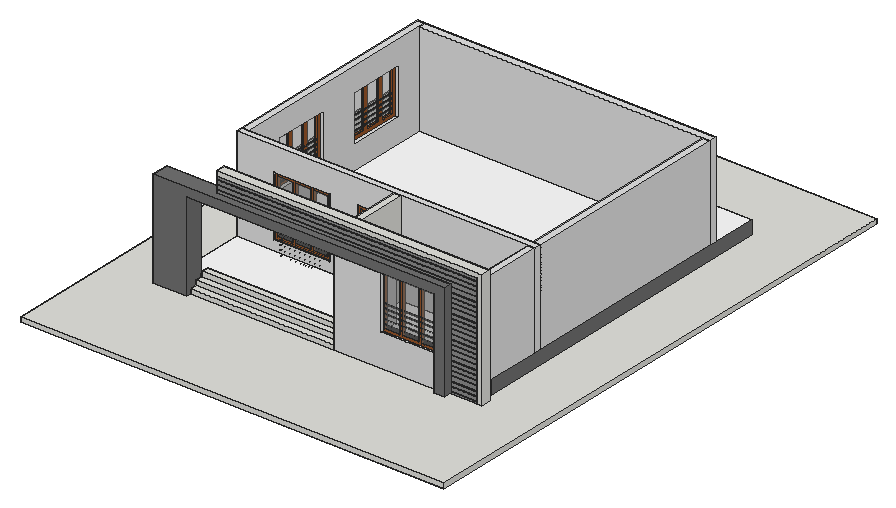
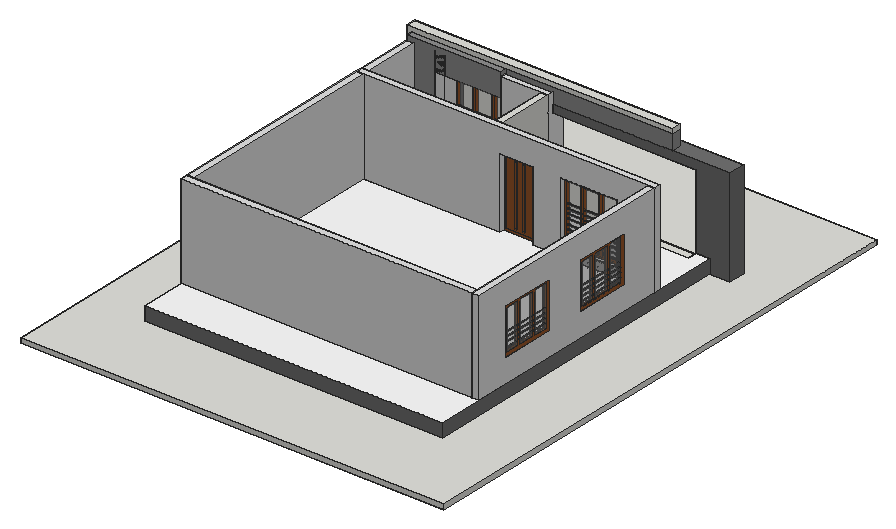
# SketchUp Ruby script. Lengths in inches.
U = 1.inch
M = Sketchup.active_model
def pt(a) = Geom::Point3d.new(a.map { |v| v * U })
def face(e, loops, mat)
  f = e.add_face(loops[0].map { |a| pt(a) })
  loops[1..].each { |l| e.add_face(l.map { |a| pt(a) }).erase! }
  f.material = f.back_material = mat if mat
  f
end
# faces: each face lists its corners as indices into pts; further lists are holes
def faces(e, pts, list, mat = nil) = list.each { |f| face(e, (f[0].is_a?(Array) ? f : [f]).map { |l| l.map { |i| pts[i] } }, mat) }
# xy, xz, yz: faces in a plane at the given z, y or x. An outline is a flat list of corners, or four numbers for a rectangle; further outlines are holes
def ring(l) = l.size == 4 ? [[l[0], l[1]], [l[2], l[1]], [l[2], l[3]], [l[0], l[3]]] : l.each_slice(2).to_a
def flat(e, list, mat, &to3) = list.each { |f| face(e, (f[0].is_a?(Array) ? f : [f]).map { |l| ring(l).map { |u, v| to3.(u, v) } }, mat) }
def xy(e, z, list, mat = nil) = flat(e, list, mat) { |x, y| [x, y, z] }
def xz(e, y, list, mat = nil) = flat(e, list, mat) { |x, z| [x, y, z] }
def yz(e, x, list, mat = nil) = flat(e, list, mat) { |y, z| [x, y, z] }
def lines(e, pts, list) = list.each { |a, b| e.add_line(pt(pts[a]), pt(pts[b])) }
# prism: a flat outline (further loops are holes) pulled along v
def prism(e, loops, v, mat = nil)
  f = face(e, loops, mat); d = Geom::Vector3d.new(v.map { |x| x * U })
  f.pushpull(f.normal.samedirection?(d) ? d.length : -d.length)
end
def box(e, o, s, mat = nil) = prism(e, [[o, [o[0] + s[0], o[1], o[2]], [o[0] + s[0], o[1] + s[1], o[2]], [o[0], o[1] + s[1], o[2]]]], [0, 0, s[2]], mat)
def at(x, y, z, deg = 0) = Geom::Transformation.translation(pt([x, y, z])) * Geom::Transformation.rotation(ORIGIN, Z_AXIS, deg.degrees)
def axes(o, x, y, z) = Geom::Transformation.new([*x, 0, *y, 0, *z, 0, *pt(o).to_a, 1])
def part(name) = M.definitions.add(name)
# library, detail: a bought-in or finely detailed component or shape, given as its bounding box
def library(name, o, s) = part(name).tap { |d| box(d.entities, o, s) }
def detail(e, o, s) = box(e.add_group.entities, o, s)
def put(e, d, t, mat = nil) = e.add_instance(d, t).tap { |i| i.material = mat if mat }
def group(e, t, mat = nil) = e.add_group.tap { |g| g.transformation = t; g.material = mat if mat }.entities
root = M.entities
M.materials.add("[Color M00]").color = [255, 255, 255]
M.materials.add("[Color M01]").color = [226, 226, 226]
M.materials.add("[Color M04]").color = [142, 142, 142]
M.materials.add("[Color M05]").color = [114, 114, 114]
M.materials.add("[Metal Silver]").color = [234, 233, 238]
M.materials.add("[Translucent Glass Gray]").color = [128, 128, 128]
M.materials["[Translucent Glass Gray]"].alpha = 0.5
M.materials.add("[Wood Cherry Original]").color = [152, 86, 42]
c1 = part("Group\#18")
prism(c1.entities,[[[0,1.11,0.71],[0,1.125,0.5625],[0,1.11,0.42],[0,1.05,0.28],[0,0.96,0.16],[0,0.84,0.08],[0,0.71,0.02],[0,0.5625,0],[0,0.42,0.02],[0,0.28,0.08],[0,0.16,0.16],[0,0.08,0.28],[0,0.02,0.42],[0,0,0.5625],[0,0.02,0.71],[0,0.08,0.84],[0,0.16,0.96],[0,0.28,1.05],[0,0.42,1.11],[0,0.5625,1.125],[0,0.71,1.11],[0,0.84,1.05],[0,0.96,0.96],[0,1.05,0.84]]],[64,0,0])
c2 = part("Group\#25")
prism(c2.entities,[[[0.28,64,0.08],[0.16,64,0.16],[0.08,64,0.28],[0.02,64,0.42],[0,64,0.5625],[0.02,64,0.71],[0.08,64,0.84],[0.16,64,0.96],[0.28,64,1.05],[0.42,64,1.11],[0.5625,64,1.125],[0.71,64,1.11],[0.84,64,1.05],[0.96,64,0.96],[1.05,64,0.84],[1.11,64,0.71],[1.125,64,0.5625],[1.11,64,0.42],[1.05,64,0.28],[0.96,64,0.16],[0.84,64,0.08],[0.71,64,0.02],[0.5625,64,0],[0.42,64,0.02]]],[0,-64,0])
c3 = part("Group\#16")
prism(c3.entities,[[[0,2,23.9375],[0,2,22.2],[0,0.74,22.2],[0,0.74,1.74],[0,2,1.74],[0,2,0],[0,0,0],[0,0,23.9375]]],[1.1875,0,0])
c4 = part("Group\#30")
prism(c4.entities,[[[0.15,64,0.15],[0.07,64,0.25],[0.02,64,0.37],[0,64,0.5],[0.02,64,0.63],[0.07,64,0.75],[0.15,64,0.85],[0.25,64,0.93],[0.37,64,0.98],[0.5,64,1],[0.63,64,0.98],[0.75,64,0.93],[0.85,64,0.85],[0.93,64,0.75],[0.98,64,0.63],[1,64,0.5],[0.98,64,0.37],[0.93,64,0.25],[0.85,64,0.15],[0.75,64,0.07],[0.63,64,0.02],[0.5,64,0],[0.37,64,0.02],[0.25,64,0.07]]],[0,-64,0])
g1 = group(root,at(0,0,0))
box(g1,[0,0,0],[542.875,691.875,6])
g2 = group(root,at(47.33,167.375,6),"[Color M05]")
xy(g2,0,[[38,-8,38,420,420,420,420,3,56,3,56,-8]])
xy(g2,18,[[38,-8,56,-8,56,3,420,3,420,420,38,420]],"[Color M00]")
xz(g2,-8,[[38,0,56,18]])
xz(g2,3,[[56,0,420,18]])
xz(g2,420,[[38,0,420,18]])
yz(g2,38,[[-8,0,420,18]])
yz(g2,56,[[-8,0,3,18]])
yz(g2,420,[[3,0,420,18]])
g3 = group(root,at(287.33,143.375,6),"[Color M01]")
xy(g3,0,[[0,0,144,24]])
xy(g3,42,[[60,0,131.9,24]])
xy(g3,114,[[0,0,60,12],[131.9,0,144,12]])
xy(g3,138,[[0,12,60,24],[131.9,12,144,24]])
xz(g3,0,[[0,0,144,0,144,114,131.9,114,131.9,42,60,42,60,114,0,114]])
xz(g3,12,[[0,114,60,138],[131.9,114,144,138]])
xz(g3,24,[[0,0,0,138,60,138,60,42,131.9,42,131.9,138,144,138,144,0]])
yz(g3,0,[[0,0,0,114,12,114,12,138,24,138,24,0]])
yz(g3,60,[[0,42,24,42,24,138,12,138,12,114,0,114]])
yz(g3,131.9,[[0,42,0,114,12,114,12,138,24,138,24,42]])
yz(g3,144,[[0,0,24,0,24,138,12,138,12,114,0,114]])
g4 = group(root,at(287.33,147.375,6),"[Color M04]")
xy(g4,0,[[144,0,180,20]])
xy(g4,2,[[144,0,180,0.5]])
xy(g4,3,[[144,0,180,0.5]])
xy(g4,8,[[144,0,180,0.5]])
xy(g4,9,[[144,0,180,0.5]])
xy(g4,14,[[144,0,180,0.5]])
xy(g4,15,[[144,0,180,0.5]])
xy(g4,20,[[144,0,180,0.5]])
xy(g4,21,[[144,0,180,0.5]])
xy(g4,26,[[144,0,180,0.5]])
xy(g4,27,[[144,0,180,0.5]])
xy(g4,32,[[144,0,180,0.5]])
xy(g4,33,[[144,0,180,0.5]])
xy(g4,38,[[144,0,180,0.5]])
xy(g4,39,[[144,0,180,0.5]])
xy(g4,44,[[144,0,180,0.5]])
xy(g4,45,[[144,0,180,0.5]])
xy(g4,50,[[144,0,180,0.5]])
xy(g4,51,[[144,0,180,0.5]])
xy(g4,56,[[144,0,180,0.5]])
xy(g4,57,[[144,0,180,0.5]])
xy(g4,62,[[144,0,180,0.5]])
xy(g4,63,[[144,0,180,0.5]])
xy(g4,68,[[144,0,180,0.5]])
xy(g4,69,[[144,0,180,0.5]])
xy(g4,74,[[144,0,180,0.5]])
xy(g4,75,[[144,0,180,0.5]])
xy(g4,80,[[144,0,180,0.5]])
xy(g4,81,[[144,0,180,0.5]])
xy(g4,86,[[144,0,180,0.5]])
xy(g4,87,[[144,0,180,0.5]])
xy(g4,92,[[144,0,180,0.5]])
xy(g4,93,[[144,0,180,0.5]])
xy(g4,98,[[144,0,180,0.5]])
xy(g4,99,[[144,0,180,0.5]])
xy(g4,104,[[144,0,180,0.5]])
xy(g4,105,[[144,0,180,0.5]])
xy(g4,110,[[144,0,180,0.5]])
xy(g4,111,[[144,0,180,0.5]])
xy(g4,114,[[0,0,0,12,60,12,60,20,144,20,144,0]])
xy(g4,116,[[0,0,180,0.5]])
xy(g4,117,[[0,0,180,0.5]])
xy(g4,122,[[0,0,180,0.5]])
xy(g4,123,[[0,0,180,0.5]])
xy(g4,125,[[-154,0,0,12]])
xy(g4,128,[[-154,0,180,0.5]])
xy(g4,129,[[-154,0,180,0.5]])
xy(g4,134,[[-154,0,180,0.5]])
xy(g4,135,[[-154,0,180,0.5]])
xy(g4,140,[[-154,0,180,0.5]])
xy(g4,141,[[-154,0,180,0.5]])
xy(g4,144,[[-154,0,180,0,180,20,60,20,60,12,-154,12]])
xz(g4,0,[[144,0,180,2],[144,3,180,8],[144,9,180,14],[144,15,180,20],[144,21,180,26],
  [144,27,180,32],[144,33,180,38],[144,39,180,44],[144,45,180,50],[144,51,180,56],
  [144,57,180,62],[144,63,180,68],[144,69,180,74],[144,75,180,80],[144,81,180,86],
  [144,87,180,92],[144,93,180,98],[144,99,180,104],[144,105,180,110],[144,111,180,111,180,116,0,116,0,114,144,114],
  [0,117,180,122],[0,123,180,123,180,128,-154,128,-154,125,0,125],[-154,129,180,134],[-154,135,180,140],[-154,141,180,144]])
xz(g4,0.5,[[144,2,180,3],[144,8,180,9],[144,14,180,15],[144,20,180,21],[144,26,180,27],
  [144,32,180,33],[144,38,180,39],[144,44,180,45],[144,50,180,51],[144,56,180,57],
  [144,62,180,63],[144,68,180,69],[144,74,180,75],[144,80,180,81],[144,86,180,87],
  [144,92,180,93],[144,98,180,99],[144,104,180,105],[144,110,180,111],[0,116,180,117],
  [0,122,180,123],[-154,128,180,129],[-154,134,180,135],[-154,140,180,141]])
xz(g4,12,[[0,114,0,125,-154,125,-154,144,60,144,60,114]])
xz(g4,20,[[144,0,144,114,60,114,60,144,180,144,180,0]])
yz(g4,-154,[[0,125,0,128,0.5,128,0.5,129,0,129,0,134,0.5,134,0.5,135,0,135,0,140,0.5,140,0.5,141,0,141,0,144,12,144,12,125]])
yz(g4,0,[[0,114,0,116,0.5,116,0.5,117,0,117,0,122,0.5,122,0.5,123,0,123,0,125,12,125,12,114]])
yz(g4,60,[[12,114,20,144]])
yz(g4,144,[[0,0,0,2,0.5,2,0.5,3,0,3,0,8,0.5,8,0.5,9,0,9,0,14,0.5,14,0.5,15,0,15,0,20,0.5,20,0.5,21,0,21,0,26,0.5,26,0.5,27,0,27,0,32,0.5,32,0.5,33,0,33,0,38,0.5,38,0.5,39,0,39,0,44,0.5,44,0.5,45,0,45,0,50,0.5,50,0.5,51,0,51,0,56,0.5,56,0.5,57,0,57,0,62,0.5,62,0.5,63,0,63,0,68,0.5,68,0.5,69,0,69,0,74,0.5,74,0.5,75,0,75,0,80,0.5,80,0.5,81,0,81,0,86,0.5,86,0.5,87,0,87,0,92,0.5,92,0.5,93,0,93,0,98,0.5,98,0.5,99,0,99,0,104,0.5,104,0.5,105,0,105,0,110,0.5,110,0.5,111,0,111,0,114,20,114,20,0]])
yz(g4,180,[[0,0,20,0,20,144,0,144,0,141,0.5,141,0.5,140,0,140,0,135,0.5,135,0.5,134,0,134,0,129,0.5,129,0.5,128,0,128,0,123,0.5,123,0.5,122,0,122,0,117,0.5,117,0.5,116,0,116,0,111,0.5,111,0.5,110,0,110,0,105,0.5,105,0.5,104,0,104,0,99,0.5,99,0.5,98,0,98,0,93,0.5,93,0.5,92,0,92,0,87,0.5,87,0.5,86,0,86,0,81,0.5,81,0.5,80,0,80,0,75,0.5,75,0.5,74,0,74,0,69,0.5,69,0.5,68,0,68,0,63,0.5,63,0.5,62,0,62,0,57,0.5,57,0.5,56,0,56,0,51,0.5,51,0.5,50,0,50,0,45,0.5,45,0.5,44,0,44,0,39,0.5,39,0.5,38,0,38,0,33,0.5,33,0.5,32,0,32,0,27,0.5,27,0.5,26,0,26,0,21,0.5,21,0.5,20,0,20,0,15,0.5,15,0.5,14,0,14,0,9,0.5,9,0.5,8,0,8,0,3,0.5,3,0.5,2,0,2]])
g5 = group(root,at(85.33,137.375,6),"[Color M05]")
xy(g5,0,[[-25,0,18,22],[334,0,348,10]])
xy(g5,114,[[18,0,18,22,202,22,202,10,334,10,334,0]])
xy(g5,125,[[-25,0,348,0,348,10,202,10,202,22,-25,22]])
xz(g5,0,[[-25,0,18,0,18,114,334,114,334,0,348,0,348,125,-25,125]])
xz(g5,10,[[334,0,334,114,202,114,202,125,348,125,348,0]])
xz(g5,22,[[-25,0,-25,125,202,125,202,114,18,114,18,0]])
yz(g5,-25,[[0,0,22,125]])
yz(g5,18,[[0,0,22,114]])
yz(g5,202,[[10,114,22,125]])
yz(g5,334,[[0,0,10,114]])
yz(g5,348,[[0,0,10,125]])
g6 = group(root,at(208.08,147.375,6))
prism(g6,[[[-74.75,0,144],[259.25,0,144],[259.25,0,0],[265.25,0,0],[265.25,0,150],[-74.75,0,150]]],[0,12,0])
g7 = group(root,at(85.33,143.375,6))
prism(g7,[[[202,27,0],[202,27,18],[202,18,18],[202,18,12],[202,9,12],[202,9,6],[202,0,6],[202,0,0]]],[-184,0,0])
put(root,c1,at(137.33,242.3125,17.07))
put(root,c1,at(137.33,242.3125,23.07))
g8 = group(root,at(47.33,239.375,24),"[Color M01]")
prism(g8,[[[194,9,0],[38,9,0],[38,9,120],[420,9,120],[420,9,0],[236,9,0],[236,9,90],[194,9,90]],[[158,9,90],[86,9,90],[86,9,12],[158,9,12]]],[0,-9,0])
g9 = group(root,at(287.33,167.375,24))
box(g9,[0,0,0],[9,72,120])
g10 = group(root,at(241.33,239.375,24),"[Wood Cherry Original]")
prism(g10,[[[42,0,90],[0,0,90],[0,0,0],[42,0,0]],[[3,0,3],[3,0,87],[39,0,87],[39,0,3]]],[0,3,0])
g11 = group(root,at(85.33,248.375,24),"[Color M01]")
prism(g11,[[[0,280.8125,0],[0,0,0],[0,0,120],[0,280.8125,120]],[[0,48,30],[0,120,30],[0,120,90],[0,48,90]],[[0,240,30],[0,240,90],[0,168,90],[0,168,30]]],[9,0,0])
g12 = group(root,at(94.33,520.1875,24),"[Color M01]")
box(g12,[0,0,0],[373,9,120])
g13 = group(root,at(458.33,248.375,24),"[Color M01]")
box(g13,[0,0,0],[9,271.8125,120])
g14 = group(root,at(458.33,167.375,24),"[Color M01]")
box(g14,[0,0,0],[9,72,120])
g15 = group(root,at(244.33,240.875,27),"[Wood Cherry Original]")
xy(g15,0,[[0,0,0,2,36,2,36,0,18.15,0,18.15,0.5,17.85,0.5,17.85,0]])
xy(g15,3,[[11.35,0,14.35,2],[21.65,0,24.65,2]])
xy(g15,24,[[2,-0.5,9.35,0],[26.65,-0.5,34,0]])
xy(g15,25,[[3,-0.5,8.35,0],[27.65,-0.5,33,0]])
xy(g15,32,[[3,-0.5,8.35,0],[27.65,-0.5,33,0]])
xy(g15,33,[[2,-0.5,9.35,0],[26.65,-0.5,34,0]])
xy(g15,42,[[2,-0.5,9.35,0],[26.65,-0.5,34,0]])
xy(g15,43,[[3,-0.5,8.35,0],[27.65,-0.5,33,0]])
xy(g15,50,[[3,-0.5,8.35,0],[27.65,-0.5,33,0]])
xy(g15,51,[[2,-0.5,9.35,0],[26.65,-0.5,34,0]])
xy(g15,60,[[2,-0.5,9.35,0],[26.65,-0.5,34,0]])
xy(g15,61,[[3,-0.5,8.35,0],[27.65,-0.5,33,0]])
xy(g15,68,[[3,-0.5,8.35,0],[27.65,-0.5,33,0]])
xy(g15,69,[[2,-0.5,9.35,0],[26.65,-0.5,34,0]])
xy(g15,81,[[11.35,0,14.35,2],[21.65,0,24.65,2]])
xy(g15,84,[[0,0,17.85,0,17.85,0.5,18.15,0.5,18.15,0,36,0,36,2,0,2]])
xz(g15,-0.5,[[[2,24,9.35,33],[3,25,8.35,32]],[[26.65,24,34,33],[27.65,25,33,32]],[[2,42,9.35,51],[3,43,8.35,50]],[[26.65,42,34,51],[27.65,43,33,50]],[[2,60,9.35,69],[3,61,8.35,68]],
  [[26.65,60,34,69],[27.65,61,33,68]]])
xz(g15,0,[[[0,0,17.85,84],[11.35,3,14.35,81],[2,60,9.35,69],[2,42,9.35,51],[2,24,9.35,33]],[[18.15,0,36,84],[21.65,3,24.65,81],[26.65,24,34,33],[26.65,42,34,51],[26.65,60,34,69]],[3,25,8.35,32],[27.65,25,33,32],[3,43,8.35,50],
  [27.65,43,33,50],[3,61,8.35,68],[27.65,61,33,68]])
xz(g15,0.5,[[17.85,0,18.15,84]])
xz(g15,2,[[[0,0,36,84],[21.65,3,24.65,81],[11.35,3,14.35,81]]])
yz(g15,0,[[0,0,2,84]])
yz(g15,2,[[-0.5,24,0,33],[-0.5,42,0,51],[-0.5,60,0,69]])
yz(g15,3,[[-0.5,25,0,32],[-0.5,43,0,50],[-0.5,61,0,68]])
yz(g15,8.35,[[-0.5,25,0,32],[-0.5,43,0,50],[-0.5,61,0,68]])
yz(g15,9.35,[[-0.5,24,0,33],[-0.5,42,0,51],[-0.5,60,0,69]])
yz(g15,11.35,[[0,3,2,81]])
yz(g15,14.35,[[0,3,2,81]])
yz(g15,17.85,[[0,0,0.5,84]])
yz(g15,18.15,[[0,0,0.5,84]])
yz(g15,21.65,[[0,3,2,81]])
yz(g15,24.65,[[0,3,2,81]])
yz(g15,26.65,[[-0.5,24,0,33],[-0.5,42,0,51],[-0.5,60,0,69]])
yz(g15,27.65,[[-0.5,25,0,32],[-0.5,43,0,50],[-0.5,61,0,68]])
yz(g15,33,[[-0.5,25,0,32],[-0.5,43,0,50],[-0.5,61,0,68]])
yz(g15,34,[[-0.5,24,0,33],[-0.5,42,0,51],[-0.5,60,0,69]])
yz(g15,36,[[0,0,2,84]])
put(root,c1,at(137.33,242.3125,29.07))
g16 = group(root,at(265.98,240.875,30),"[Translucent Glass Gray]")
xz(g16,0,[[0,0,3,78]])
g17 = group(root,at(255.68,240.875,30),"[Translucent Glass Gray]")
xz(g17,0,[[0,0,3,78]])
put(root,c1,at(137.33,242.3125,35.07))
g18 = group(root,at(133.33,241.375,36),"[Wood Cherry Original]")
prism(g18,[[[72,0,78],[0,0,78],[0,0,0],[72,0,0]],[[46,0,4],[26,0,4],[26,0,74],[46,0,74]],[[22,0,74],[22,0,4],[4,0,4],[4,0,74]],[[50,0,4],[50,0,74],[68,0,74],[68,0,4]]],[0,3,0])
g19 = group(root,at(183.33,241.375,40),"[Translucent Glass Gray]")
xz(g19,0,[[0,0,18,70]])
g20 = group(root,at(159.33,241.375,40),"[Translucent Glass Gray]")
xz(g20,0,[[0,0,20,70]])
g21 = group(root,at(137.33,241.375,40),"[Translucent Glass Gray]")
xz(g21,0,[[0,0,18,70]])
put(root,c1,at(137.33,242.3125,41.07))
put(root,c1,at(137.33,242.3125,47.07))
g22 = group(root,at(347.33,146.375,48),"[Wood Cherry Original]")
prism(g22,[[[72,3,0],[0,3,0],[0,3,72],[72,3,72]],[[46,3,3],[46,3,69],[26,3,69],[26,3,3]],[[22,3,3],[22,3,69],[3,3,69],[3,3,3]],[[69,3,69],[50,3,69],[50,3,3],[69,3,3]]],[0,-3,0])
g23 = group(root,at(397.33,146.375,51),"[Translucent Glass Gray]")
xz(g23,0,[[0,0,19,66]])
g24 = group(root,at(373.33,146.375,51),"[Translucent Glass Gray]")
xz(g24,0,[[0,0,20,66]])
g25 = group(root,at(350.33,146.375,51),"[Translucent Glass Gray]")
xz(g25,0,[[0,0,19,66]])
put(root,c1,at(137.33,242.3125,53.07))
g26 = group(root,at(86.33,296.375,54),"[Wood Cherry Original]")
prism(g26,[[[0,72,0],[0,0,0],[0,0,60],[0,72,60]],[[0,26,4],[0,46,4],[0,46,56],[0,26,56]],[[0,22,4],[0,22,56],[0,4,56],[0,4,4]],[[0,50,56],[0,50,4],[0,68,4],[0,68,56]]],[3,0,0])
g27 = group(root,at(86.33,416.375,54),"[Wood Cherry Original]")
prism(g27,[[[0,0,60],[0,72,60],[0,72,0],[0,0,0]],[[0,26,56],[0,26,4],[0,46,4],[0,46,56]],[[0,68,56],[0,50,56],[0,50,4],[0,68,4]],[[0,4,4],[0,22,4],[0,22,56],[0,4,56]]],[3,0,0])
g28 = group(root,at(352.33,147.5,54.5))
prism(g28,[[[64,0.11,0.64],[64,0.05,0.5625],[64,0.01,0.47],[64,0,0.375],[64,0.01,0.28],[64,0.05,0.1875],[64,0.11,0.11],[64,0.1875,0.05],[64,0.28,0.01],[64,0.375,0],[64,0.47,0.01],[64,0.5625,0.05],[64,0.64,0.11],[64,0.7,0.1875],[64,0.74,0.28],[64,0.75,0.375],[64,0.74,0.47],[64,0.7,0.5625],[64,0.64,0.64],[64,0.5625,0.7],[64,0.47,0.74],[64,0.375,0.75],[64,0.28,0.74],[64,0.1875,0.7]]],[-69,0,0])
put(root,c2,at(87.27,300.375,56.45))
g29 = group(root,at(86.33,300.375,58),"[Translucent Glass Gray]")
yz(g29,0,[[0,0,18,52]])
g30 = group(root,at(86.33,322.375,58),"[Translucent Glass Gray]")
yz(g30,0,[[0,0,20,52]])
g31 = group(root,at(86.33,346.375,58),"[Translucent Glass Gray]")
yz(g31,0,[[0,0,18,52]])
g32 = group(root,at(86.33,420.375,58),"[Translucent Glass Gray]")
yz(g32,0,[[0,0,18,52]])
g33 = group(root,at(86.33,442.375,58),"[Translucent Glass Gray]")
yz(g33,0,[[0,0,20,52]])
g34 = group(root,at(86.33,466.375,58),"[Translucent Glass Gray]")
yz(g34,0,[[0,0,18,52]])
put(root,c3,at(259.73,238.875,58.14),"[Metal Silver]")
put(root,c3,at(263.54,238.875,58.14),"[Metal Silver]")
put(root,c1,at(137.33,242.3125,59.07))
g35 = group(root,at(352.33,147.5,60.5))
prism(g35,[[[64,0.11,0.64],[64,0.05,0.5625],[64,0.01,0.47],[64,0,0.375],[64,0.01,0.28],[64,0.05,0.1875],[64,0.11,0.11],[64,0.1875,0.05],[64,0.28,0.01],[64,0.375,0],[64,0.47,0.01],[64,0.5625,0.05],[64,0.64,0.11],[64,0.7,0.1875],[64,0.74,0.28],[64,0.75,0.375],[64,0.74,0.47],[64,0.7,0.5625],[64,0.64,0.64],[64,0.5625,0.7],[64,0.47,0.74],[64,0.375,0.75],[64,0.28,0.74],[64,0.1875,0.7]]],[-69,0,0])
put(root,c2,at(87.27,300.375,62.45))
put(root,c4,at(87.33,420.375,62.78))
put(root,c1,at(137.33,242.3125,65.07))
g36 = group(root,at(352.33,147.5,66.5))
prism(g36,[[[64,0.11,0.64],[64,0.05,0.5625],[64,0.01,0.47],[64,0,0.375],[64,0.01,0.28],[64,0.05,0.1875],[64,0.11,0.11],[64,0.1875,0.05],[64,0.28,0.01],[64,0.375,0],[64,0.47,0.01],[64,0.5625,0.05],[64,0.64,0.11],[64,0.7,0.1875],[64,0.74,0.28],[64,0.75,0.375],[64,0.74,0.47],[64,0.7,0.5625],[64,0.64,0.64],[64,0.5625,0.7],[64,0.47,0.74],[64,0.375,0.75],[64,0.28,0.74],[64,0.1875,0.7]]],[-69,0,0])
put(root,c2,at(87.27,300.375,68.45))
put(root,c4,at(87.33,420.375,68.78))
put(root,c1,at(137.33,242.3125,71.07))
g37 = group(root,at(352.33,147.5,72.5))
prism(g37,[[[64,0.11,0.64],[64,0.05,0.5625],[64,0.01,0.47],[64,0,0.375],[64,0.01,0.28],[64,0.05,0.1875],[64,0.11,0.11],[64,0.1875,0.05],[64,0.28,0.01],[64,0.375,0],[64,0.47,0.01],[64,0.5625,0.05],[64,0.64,0.11],[64,0.7,0.1875],[64,0.74,0.28],[64,0.75,0.375],[64,0.74,0.47],[64,0.7,0.5625],[64,0.64,0.64],[64,0.5625,0.7],[64,0.47,0.74],[64,0.375,0.75],[64,0.28,0.74],[64,0.1875,0.7]]],[-69,0,0])
put(root,c2,at(87.27,300.375,74.45))
put(root,c4,at(87.33,420.375,74.78))
put(root,c1,at(137.33,242.3125,77.07))
g38 = group(root,at(352.33,147.5,78.5))
prism(g38,[[[64,0.11,0.64],[64,0.05,0.5625],[64,0.01,0.47],[64,0,0.375],[64,0.01,0.28],[64,0.05,0.1875],[64,0.11,0.11],[64,0.1875,0.05],[64,0.28,0.01],[64,0.375,0],[64,0.47,0.01],[64,0.5625,0.05],[64,0.64,0.11],[64,0.7,0.1875],[64,0.74,0.28],[64,0.75,0.375],[64,0.74,0.47],[64,0.7,0.5625],[64,0.64,0.64],[64,0.5625,0.7],[64,0.47,0.74],[64,0.375,0.75],[64,0.28,0.74],[64,0.1875,0.7]]],[-69,0,0])
put(root,c2,at(87.27,300.375,80.45))
put(root,c4,at(87.33,420.375,80.78))
put(root,c1,at(137.33,242.3125,83.07))
